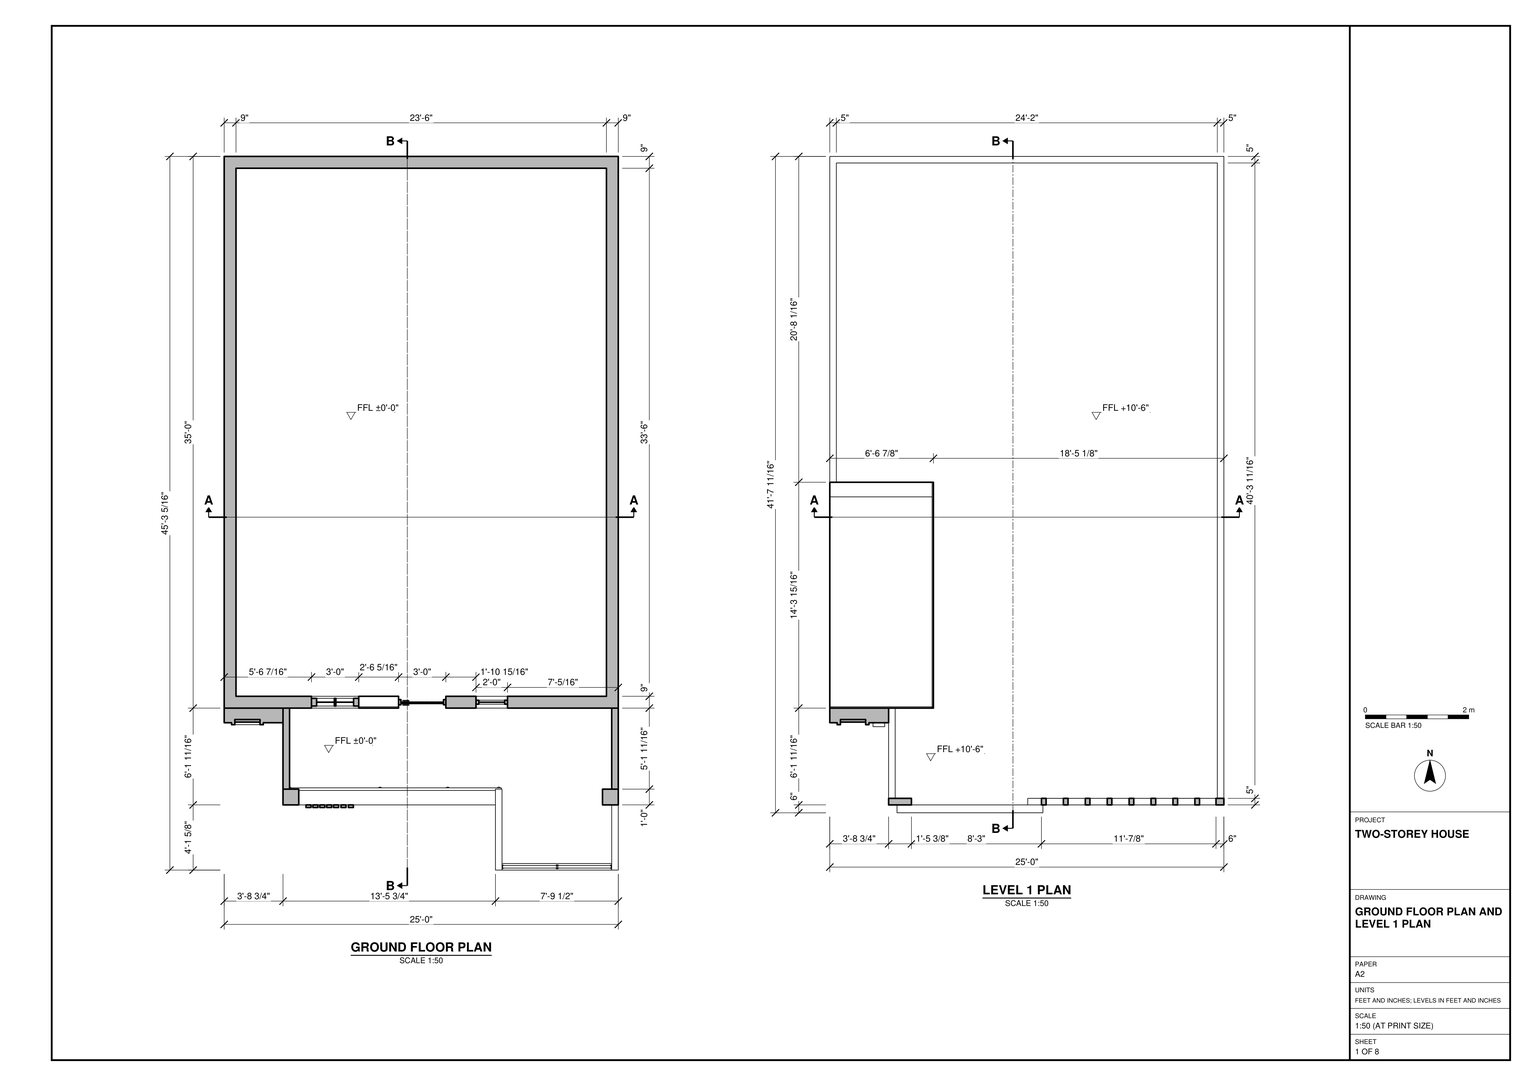
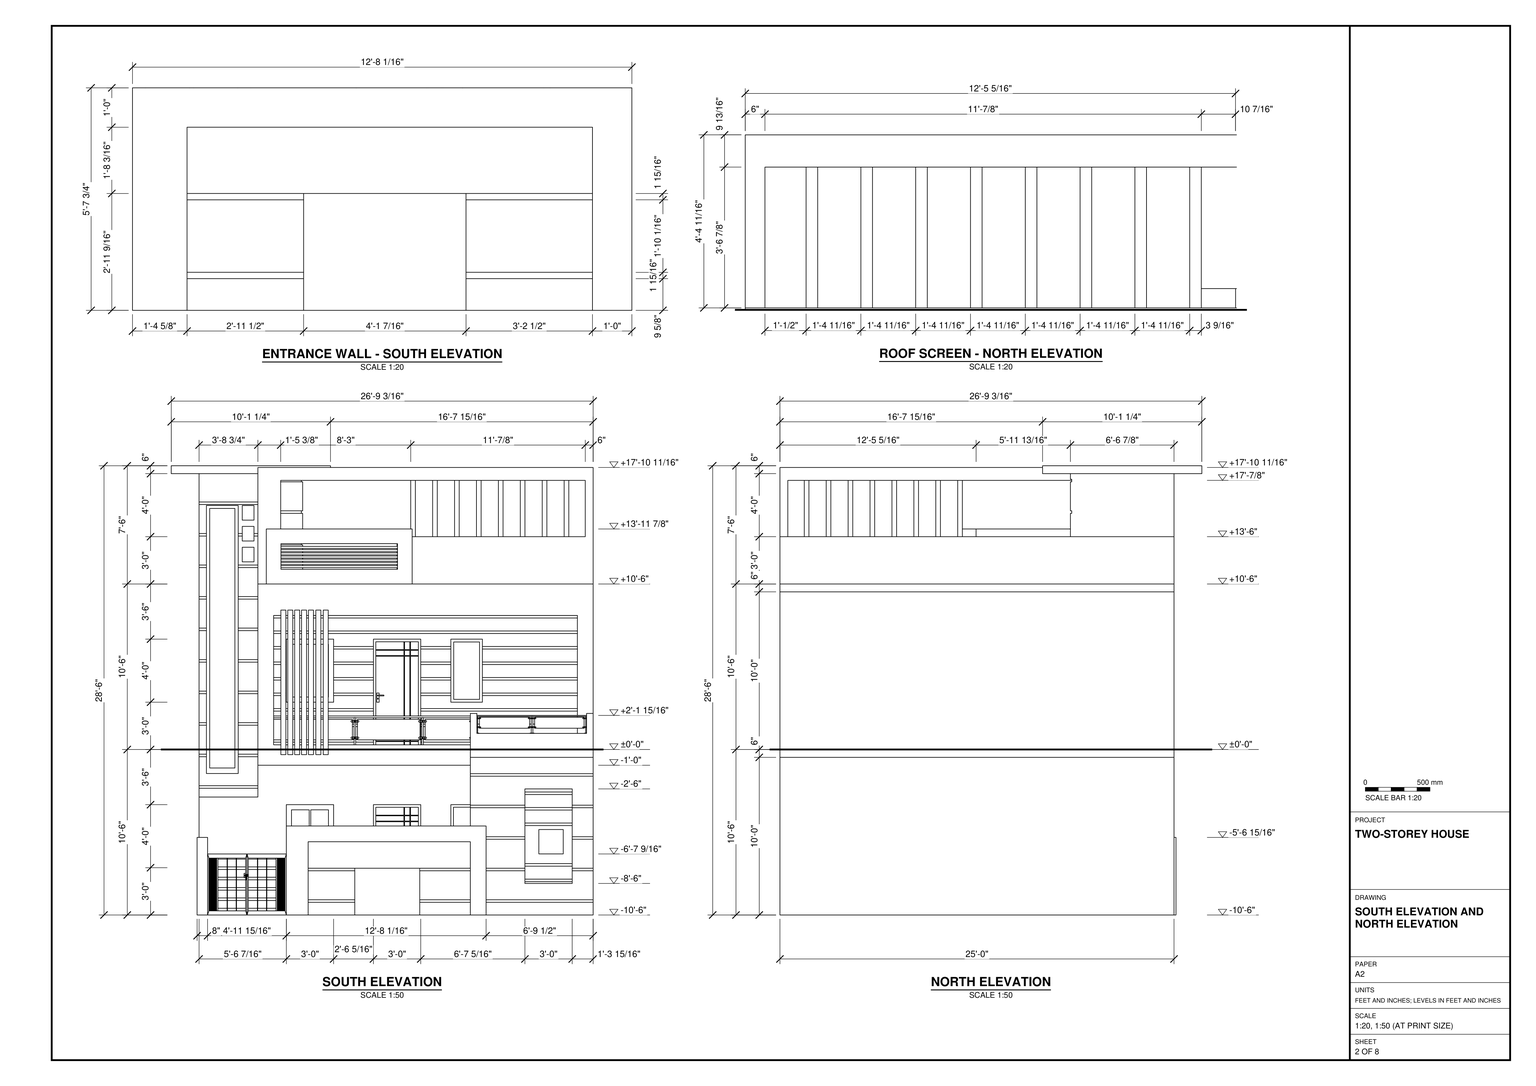
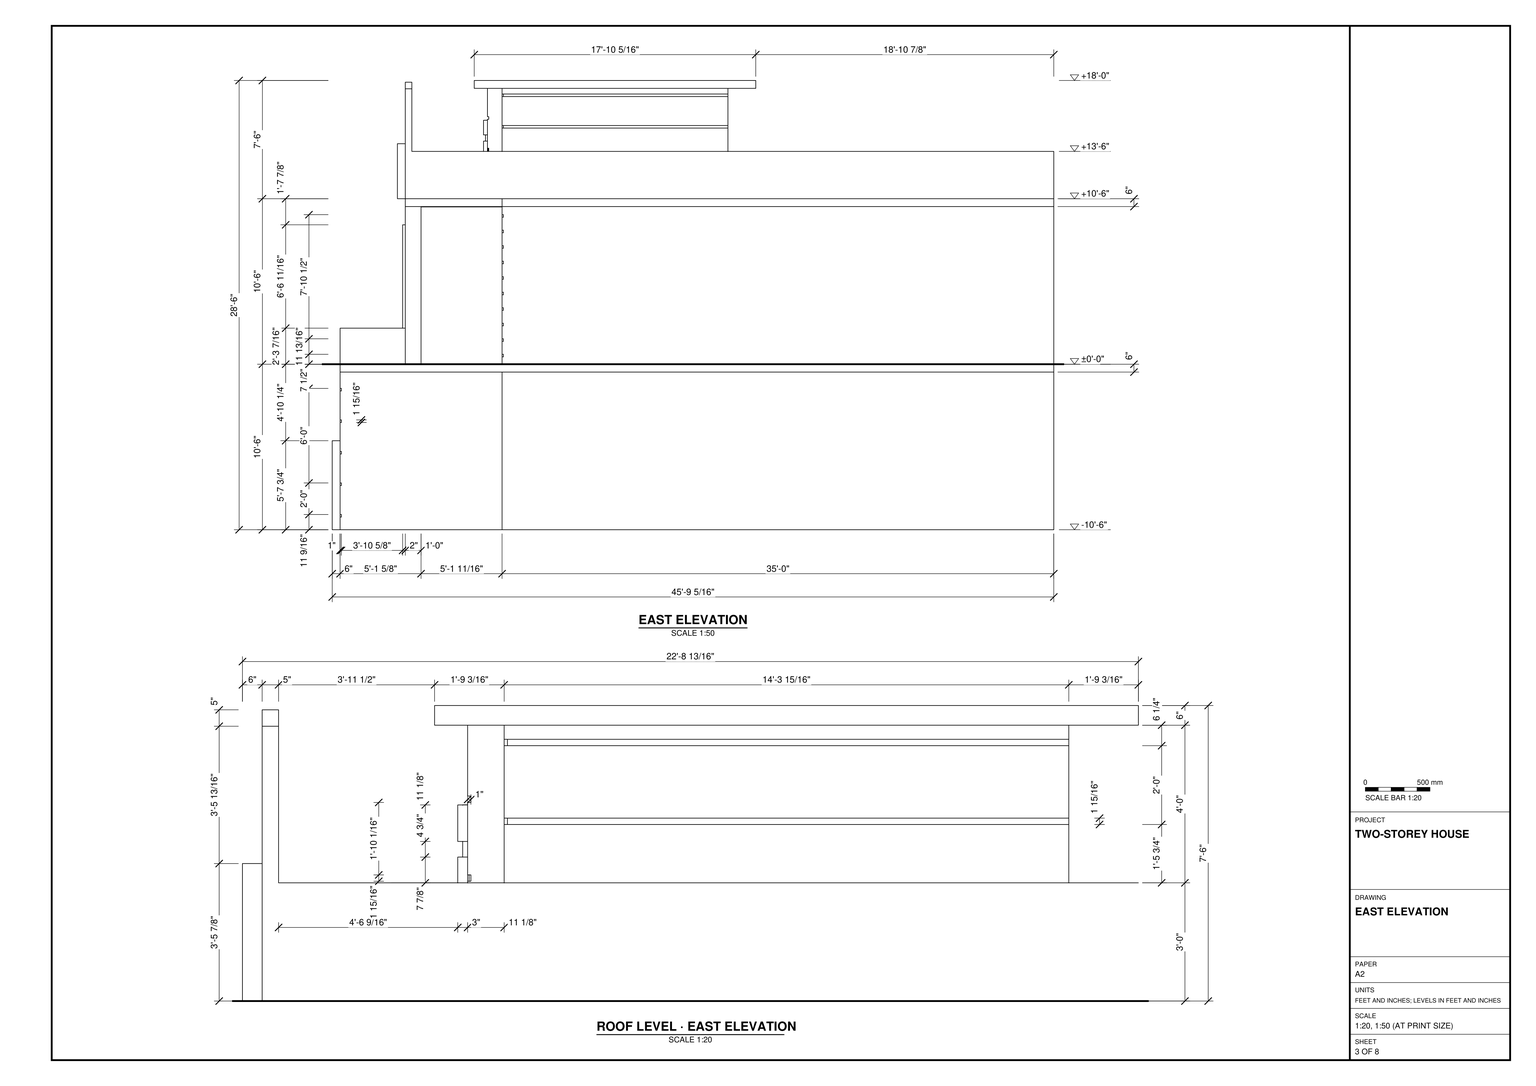
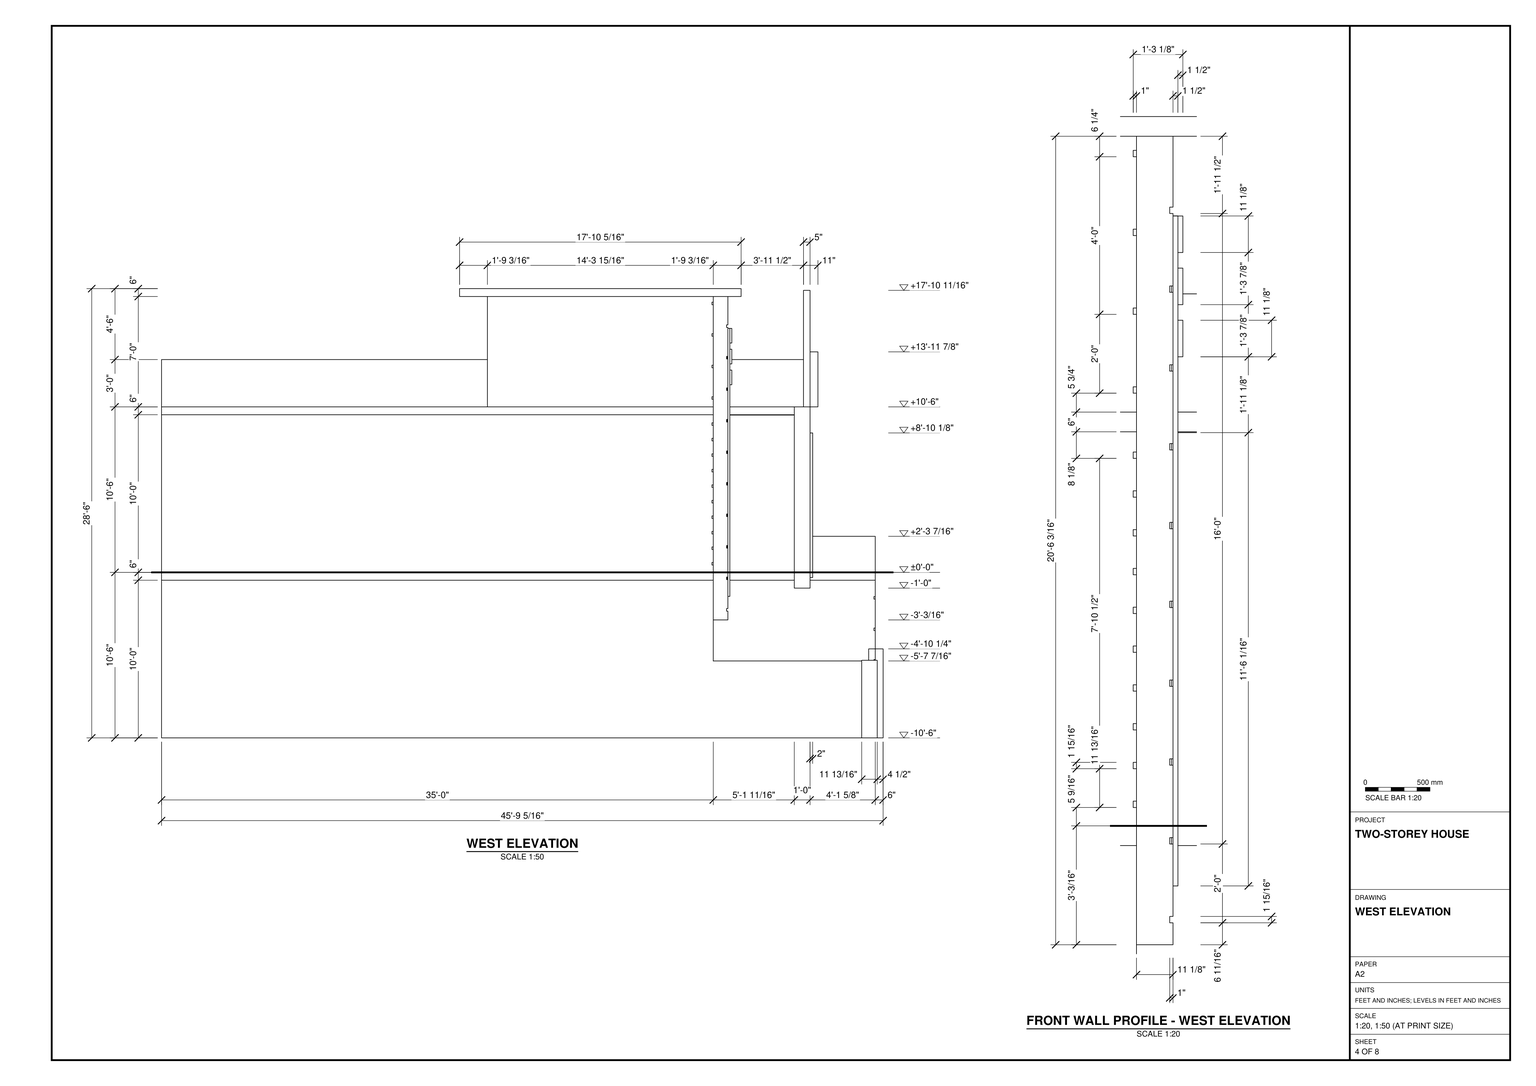
Build the two-storey house in SketchUp from task_files/diagram_01.pdf. Work in feet and inches. Set the ground floor at ±0'-0" and the next storey at +10'-6". The overall model, including the front projections and roof overhang, is 26'-9 3/16" wide, 45'-9 5/16" deep and 28'-6" high.

Start with the 25'-0" by 35'-0" rectangular ground-floor block. Use the wall thicknesses shown in plan and the slab thicknesses shown in elevation. Build the stepped south frontage around the recessed door and window openings. At the lower entrance, place the gate beside the broad framed entrance wall. Above it, model the balcony with its low railing, the horizontal bands on the wall behind it, the tall narrow panel at the left and the row of vertical fins. Follow the plans and elevations for the flat roof, low terrace parapet, raised canopy and roof screen, distinguishing the upright screen members from the horizontal slats.

Use separate groups or components for the walls, slabs, roof and each furniture or joinery piece shown. Use components for repeated parts. Any decor or loose items shown may be represented by suitable library components. Save one SketchUp model as output_files/two_storey_house_with_a_screened_roof_terrace.skp.

# SketchUp Ruby script. Lengths in inches.
U = 1.inch
M = Sketchup.active_model
def pt(a) = Geom::Point3d.new(a.map { |v| v * U })
def face(e, loops, mat)
  f = e.add_face(loops[0].map { |a| pt(a) })
  loops[1..].each { |l| e.add_face(l.map { |a| pt(a) }).erase! }
  f.material = f.back_material = mat if mat
  f
end
# faces: each face lists its corners as indices into pts; further lists are holes
def faces(e, pts, list, mat = nil) = list.each { |f| face(e, (f[0].is_a?(Array) ? f : [f]).map { |l| l.map { |i| pts[i] } }, mat) }
# xy, xz, yz: faces in a plane at the given z, y or x. An outline is a flat list of corners, or four numbers for a rectangle; further outlines are holes
def ring(l) = l.size == 4 ? [[l[0], l[1]], [l[2], l[1]], [l[2], l[3]], [l[0], l[3]]] : l.each_slice(2).to_a
def flat(e, list, mat, &to3) = list.each { |f| face(e, (f[0].is_a?(Array) ? f : [f]).map { |l| ring(l).map { |u, v| to3.(u, v) } }, mat) }
def xy(e, z, list, mat = nil) = flat(e, list, mat) { |x, y| [x, y, z] }
def xz(e, y, list, mat = nil) = flat(e, list, mat) { |x, z| [x, y, z] }
def yz(e, x, list, mat = nil) = flat(e, list, mat) { |y, z| [x, y, z] }
def lines(e, pts, list) = list.each { |a, b| e.add_line(pt(pts[a]), pt(pts[b])) }
# prism: a flat outline (further loops are holes) pulled along v
def prism(e, loops, v, mat = nil)
  f = face(e, loops, mat); d = Geom::Vector3d.new(v.map { |x| x * U })
  f.pushpull(f.normal.samedirection?(d) ? d.length : -d.length)
end
def box(e, o, s, mat = nil) = prism(e, [[o, [o[0] + s[0], o[1], o[2]], [o[0] + s[0], o[1] + s[1], o[2]], [o[0], o[1] + s[1], o[2]]]], [0, 0, s[2]], mat)
def at(x, y, z, deg = 0) = Geom::Transformation.translation(pt([x, y, z])) * Geom::Transformation.rotation(ORIGIN, Z_AXIS, deg.degrees)
def axes(o, x, y, z) = Geom::Transformation.new([*x, 0, *y, 0, *z, 0, *pt(o).to_a, 1])
def part(name) = M.definitions.add(name)
# library, detail: a bought-in or finely detailed component or shape, given as its bounding box
def library(name, o, s) = part(name).tap { |d| box(d.entities, o, s) }
def detail(e, o, s) = box(e.add_group.entities, o, s)
def put(e, d, t, mat = nil) = e.add_instance(d, t).tap { |i| i.material = mat if mat }
def group(e, t, mat = nil) = e.add_group.tap { |g| g.transformation = t; g.material = mat if mat }.entities
root = M.entities
M.materials.add("[Blacktop Old 02]").color = [143, 145, 145]
M.materials.add("[Color A01]").color = [255, 204, 204]
M.materials.add("[Color B03]").color = [255, 140, 101]
M.materials.add("[Color C03]").color = [255, 178, 101]
M.materials.add("[Color E05]").color = [255, 255, 0]
M.materials.add("[Color G02]").color = [153, 255, 153]
M.materials.add("[Color H06]").color = [0, 204, 204]
M.materials.add("[Color M00]").color = [255, 255, 255]
M.materials.add("[Color M05]").color = [114, 114, 114]
M.materials.add("[Color M09]").color = [0, 0, 0]
M.materials.add("[Formica Beige]").color = [211, 187, 149]
M.materials.add("[Translucent Glass Blue]").color = [100, 149, 237]
M.materials["[Translucent Glass Blue]"].alpha = 0.5
M.materials.add("[Wood Cherry Original]").color = [152, 86, 42]
c1 = library("Untitled",[0,0,0],[36,4.39,84])
c2 = library("Untitled\#1",[131.66,19.68,0],[2.41,197.25,46.46])
c3 = part("Group4\#2")
xy(c3.entities,0,[[-14.0625,-20.0625,-0.59,20.0625],[0.59,-20.0625,14.0625,20.0625]])
c4 = part("Group3\#1")
prism(c4.entities,[[[-18,24,0],[18,24,0],[18,-24,0],[-18,-24,0]],[[0.59,20.0625,0],[0.59,-20.0625,0],[14.0625,-20.0625,0],[14.0625,20.0625,0]],[[-0.59,20.0625,0],[-14.0625,20.0625,0],[-14.0625,-20.0625,0],[-0.59,-20.0625,0]]],[0,0,5.875])
put(c4.entities,c3,at(0,0,2.9375),"[Translucent Glass Blue]")
c5 = part("Group\#15")
box(c5.entities,[0,0,0],[3.8125,110.0625,2],"[Wood Cherry Original]")
c6 = part("Group\#6")
box(c6.entities,[0,0,0],[8.9375,11.125,3])
c7 = part("Group22\#1")
xy(c7.entities,126,[[295,-61.6875,300,0]])
xy(c7.entities,246,[[295,-61.6875,300,0]])
xz(c7.entities,-61.6875,[[295,126,300,246]])
xz(c7.entities,0,[[295,126,300,246]])
yz(c7.entities,295,[[-61.6875,126,0,246]])
yz(c7.entities,300,[[-61.6875,126,0,246]],"[Color M00]")
c8 = part("Group21\#1")
xy(c8.entities,126,[[206.5,-123.3125,211.5,-61.6875],[211.5,-123.3125,211.5,-118.3125,295,-118.3125,295,-73.6875,300,-73.6875,300,-123.3125]])
xy(c8.entities,138.25,[[211.5,-123.3125,295,-118.3125]])
xy(c8.entities,153.4375,[[206.5,-123.3125,211.5,-61.6875],[295,-123.3125,300,-73.6875]])
xz(c8.entities,-123.3125,[[206.5,126,300,126,300,153.4375,295,153.4375,295,138.25,211.5,138.25,211.5,153.4375,206.5,153.4375]])
xz(c8.entities,-118.3125,[[211.5,126,295,138.25]])
xz(c8.entities,-73.6875,[[295,126,300,153.4375]])
xz(c8.entities,-61.6875,[[206.5,126,211.5,153.4375]])
yz(c8.entities,206.5,[[-123.3125,126,-61.6875,153.4375]])
yz(c8.entities,211.5,[[-118.3125,126,-61.6875,153.4375],[-123.3125,138.25,-118.3125,153.4375]])
yz(c8.entities,295,[[-118.3125,126,-118.3125,138.25,-123.3125,138.25,-123.3125,153.4375,-73.6875,153.4375,-73.6875,126]])
yz(c8.entities,300,[[-123.3125,126,-73.6875,153.4375]])
c9 = part("Group22\#2")
box(c9.entities,[295,-61.6875,126],[5,61.6875,120])
c10 = library("Group\#9",[0,0,0],[87.4375,3.15,36.98])
c11 = library("Group\#10",[0,0,0],[163.16,3.15,36.98])
c12 = part("Group\#16")
box(c12.entities,[0,0,0],[2.53,1.5625,88.69])
c13 = part("Group\#17")
box(c13.entities,[0,0,0],[3.53,5,42.875])
c14 = part("Group31\#1")
xy(c14.entities,252,[[150.6875,-73.6875,150.6875,-68.6875,295,-68.6875,295,415,5,415,5,171.9375,0,171.9375,0,420,300,420,300,-73.6875],[44.78,-73.6875,62.15,-68.6875]])
xy(c14.entities,252,[[51.1875,-79.6875,150.6875,-73.6875],[150.6875,-79.6875,162.23,-73.6875]],"[Color G02]")
xy(c14.entities,263.17,[[150.6875,-79.6875,151.05,-73.6875]])
xy(c14.entities,263.17,[[62.36,-79.6875,150.6875,-73.6875]],"[Color G02]")
xy(c14.entities,282.7,[[62.36,-79.6875,151.05,-73.6875]],"[Color G02]")
xy(c14.entities,288,[[150.6875,-73.6875,277.9375,-68.6875],[281.47,-73.6875,294,-68.6875]])
xy(c14.entities,288,[[295,-68.6875,300,-68.6875,300,420,0,420,0,171.9375,5,171.9375,5,415,295,415]],"[Color M00]")
xy(c14.entities,293.875,[[51.1875,-79.6875,162.23,-73.6875]],"[Color G02]")
xy(c14.entities,330.875,[[62.15,-73.6875,294,-68.6875]])
xy(c14.entities,340.6875,[[44.78,-73.6875,300,-68.6875]])
xz(c14.entities,-79.6875,[[[51.1875,252,162.23,293.875],[62.36,263.17,151.05,282.7]]],"[Color G02]")
xz(c14.entities,-73.6875,[[44.78,252,51.1875,252,51.1875,293.875,62.15,293.875,62.15,330.875,294,330.875,294,288,162.23,288,162.23,252,300,252,300,340.6875,44.78,340.6875],[51.1875,252,62.15,293.875],[150.6875,252,150.6875,263.17,151.05,263.17,151.05,282.7,150.6875,282.7,150.6875,288,162.23,288,162.23,252],[150.6875,263.17,151.05,282.7],[150.6875,288,162.23,293.875]])
xz(c14.entities,-73.6875,[[62.15,252,62.15,293.875,150.6875,293.875,150.6875,282.7,62.36,282.7,62.36,263.17,150.6875,263.17,150.6875,252]],"[Color G02]")
xz(c14.entities,-68.6875,[[44.78,252,44.78,340.6875,300,340.6875,300,288,294,288,294,330.875,62.15,330.875,62.15,252]])
xz(c14.entities,-68.6875,[[150.6875,252,295,288]],"[Formica Beige]")
xz(c14.entities,171.9375,[[0,252,5,288]])
xz(c14.entities,415,[[5,252,295,288]],"[Color M00]")
xz(c14.entities,420,[[0,252,300,288]],"[Color M00]")
yz(c14.entities,0,[[171.9375,252,420,288]],"[Color M00]")
yz(c14.entities,5,[[171.9375,252,415,288]],"[Color M00]")
yz(c14.entities,44.78,[[-73.6875,252,-68.6875,340.6875]])
yz(c14.entities,51.1875,[[-79.6875,252,-73.6875,293.875]],"[Color G02]")
yz(c14.entities,62.15,[[-73.6875,252,-68.6875,330.875]])
yz(c14.entities,62.36,[[-79.6875,263.17,-73.6875,282.7]],"[Color G02]")
yz(c14.entities,150.6875,[[-73.6875,252,-68.6875,288]])
yz(c14.entities,151.05,[[-79.6875,263.17,-73.6875,282.7]],"[Color G02]")
yz(c14.entities,162.23,[[-79.6875,252,-73.6875,293.875]],"[Color G02]")
yz(c14.entities,294,[[-73.6875,288,-68.6875,330.875]])
yz(c14.entities,295,[[-68.6875,252,415,288]],"[Color M00]")
yz(c14.entities,300,[[-73.6875,335.6875,-68.6875,340.6875]])
yz(c14.entities,300,[[-73.6875,252,420,252,420,288,-68.6875,288,-68.6875,335.6875,-73.6875,335.6875]],"[Color M00]")
p = [[295,-73.6875,335.6875],[295,-68.6875,335.6875]]
lines(c14.entities,p,[[0,1]])
put(c14.entities,c12,axes([62.36,-78.14,279.05],[0,1,0],[0,0,1],[1,0,0]),"[Color M05]")
put(c14.entities,c12,axes([62.36,-78.14,276.61],[0,1,0],[0,0,1],[1,0,0]),"[Color M05]")
put(c14.entities,c12,axes([62.36,-78.14,274.17],[0,1,0],[0,0,1],[1,0,0]),"[Color M05]")
put(c14.entities,c12,axes([62.36,-78.14,271.74],[0,1,0],[0,0,1],[1,0,0]),"[Color M05]")
put(c14.entities,c12,axes([62.36,-78.14,269.3],[0,1,0],[0,0,1],[1,0,0]),"[Color M05]")
put(c14.entities,c12,axes([62.36,-78.14,266.86],[0,1,0],[0,0,1],[1,0,0]),"[Color M05]")
put(c14.entities,c12,axes([62.36,-78.14,264.42],[0,1,0],[0,0,1],[1,0,0]),"[Color M05]")
put(c14.entities,c12,axes([62.36,-78.14,259.55],[0,1,0],[0,0,1],[1,0,0]))
put(c14.entities,c12,axes([62.36,-78.14,257.11],[0,1,0],[0,0,1],[1,0,0]))
put(c14.entities,c13,at(277.9375,-73.6875,288))
put(c14.entities,c13,at(161.125,-73.6875,288))
put(c14.entities,c13,at(177.8125,-73.6875,288))
put(c14.entities,c13,at(194.5,-73.6875,288))
put(c14.entities,c13,at(211.1875,-73.6875,288))
put(c14.entities,c13,at(227.875,-73.6875,288))
put(c14.entities,c13,at(244.5625,-73.6875,288))
put(c14.entities,c13,at(261.25,-73.6875,288))
c15 = part("Group32\#1")
prism(c15.entities,[[[44.78,0,288.02],[44.78,0,252.02],[44.78,-68.6875,252],[44.78,-68.6875,288]]],[5,0,0])
xy(root,36,[[212.875,132.3125,236.875,135.3125]])
xy(root,37.96,[[214.83,132.3125,234.92,133.8125],[214.83,133.8125,234.92,135.3125]],"[Color M09]")
xy(root,82.04,[[214.83,132.3125,234.92,133.8125],[214.83,133.8125,234.92,135.3125]],"[Color M09]")
xy(root,84,[[212.875,132.3125,236.875,135.3125]])
xy(root,89.79,[[21.1875,118.1875,65.96,129.3125]])
xy(root,96.48,[[21.1875,118.1875,65.96,119.1875]],"[Color G02]")
xy(root,98.42,[[21.1875,118.1875,65.96,119.1875]],"[Color G02]")
xy(root,107.71,[[26.79,116.6875,50.99,118.1875]])
xy(root,111.9,[[29.3,116.6875,48.48,118.66],[29.3,118.66,48.48,120.625]])
xy(root,120.48,[[21.1875,118.1875,26.79,119.1875],[50.99,118.1875,65.96,119.1875]],"[Color G02]")
xy(root,122.42,[[21.1875,118.1875,26.79,119.1875],[50.99,118.1875,65.96,119.1875]],"[Color G02]")
xy(root,144.48,[[21.1875,118.1875,26.79,119.1875],[50.99,118.1875,65.96,119.1875]],"[Color G02]")
xy(root,146.42,[[21.1875,118.1875,26.79,119.1875],[50.99,118.1875,65.96,119.1875]],"[Color G02]")
xy(root,162,[[212.875,132.3125,236.875,135.3125]])
xy(root,164.17,[[215.04,132.3125,234.71,133.8125],[215.04,133.8125,234.71,135.3125]],"[Color M09]")
xy(root,168.48,[[21.1875,118.1875,26.79,119.1875],[50.99,118.1875,65.96,119.1875]],"[Color G02]")
xy(root,170.42,[[21.1875,118.1875,26.79,119.1875],[50.99,118.1875,65.96,119.1875]],"[Color G02]")
xy(root,192.48,[[21.1875,118.1875,26.79,119.1875],[50.99,118.1875,65.96,119.1875]],"[Color G02]")
xy(root,194.42,[[21.1875,118.1875,26.79,119.1875],[50.99,118.1875,65.96,119.1875]],"[Color G02]")
xy(root,207.83,[[215.04,132.3125,234.71,133.8125],[215.04,133.8125,234.71,135.3125]],"[Color M09]")
xy(root,210,[[212.875,132.3125,236.875,135.3125]])
xy(root,216.48,[[21.1875,118.1875,26.79,119.1875],[50.99,118.1875,65.96,119.1875]],"[Color G02]")
xy(root,218.42,[[21.1875,118.1875,26.79,119.1875],[50.99,118.1875,65.96,119.1875]],"[Color G02]")
xy(root,240.48,[[21.1875,118.1875,26.79,119.1875],[50.99,118.1875,65.96,119.1875]],"[Color G02]")
xy(root,242.42,[[21.1875,118.1875,26.79,119.1875],[50.99,118.1875,65.96,119.1875]],"[Color G02]")
xy(root,264.48,[[21.1875,118.1875,26.79,119.1875],[50.99,118.1875,65.96,119.1875]],"[Color G02]")
xy(root,266.42,[[21.1875,118.1875,26.79,119.1875],[50.99,118.1875,65.96,119.1875]],"[Color G02]")
xy(root,288.48,[[21.1875,118.1875,26.79,119.1875],[50.99,118.1875,65.96,119.1875]],"[Color G02]")
xy(root,290.42,[[21.1875,118.1875,26.79,119.1875],[50.99,118.1875,65.96,119.1875]],"[Color G02]")
xy(root,309.52,[[29.3,116.6875,48.48,118.66],[29.3,118.66,48.48,120.625]])
xy(root,311.76,[[26.79,116.6875,50.99,118.1875]])
xy(root,312.48,[[21.1875,118.1875,65.96,119.1875]],"[Color G02]")
xy(root,314.42,[[21.1875,118.1875,65.96,119.1875]],"[Color G02]")
xy(root,336,[[21.1875,118.1875,65.96,129.3125]],"[Color G02]")
xz(root,116.6875,[[[26.79,107.71,50.99,311.76],[29.3,111.9,48.48,309.52]]])
xz(root,118.1875,[[21.1875,89.79,65.96,96.48],[21.1875,98.42,65.96,98.42,65.96,120.48,50.99,120.48,50.99,107.71,26.79,107.71,26.79,120.48,21.1875,120.48],[21.1875,122.42,26.79,144.48],[50.99,122.42,65.96,144.48],[21.1875,146.42,26.79,168.48],
  [50.99,146.42,65.96,168.48],[21.1875,170.42,26.79,192.48],[50.99,170.42,65.96,192.48],[21.1875,194.42,26.79,216.48],[50.99,194.42,65.96,216.48],
  [21.1875,218.42,26.79,240.48],[50.99,218.42,65.96,240.48],[21.1875,242.42,26.79,264.48],[50.99,242.42,65.96,264.48],[21.1875,266.42,26.79,288.48],
  [50.99,266.42,65.96,288.48],[21.1875,290.42,26.79,290.42,26.79,311.76,50.99,311.76,50.99,290.42,65.96,290.42,65.96,312.48,21.1875,312.48],[21.1875,314.42,65.96,336]],"[Color G02]")
xz(root,118.66,[[29.3,111.9,48.48,309.52]],"[Translucent Glass Blue]")
xz(root,119.1875,[[21.1875,96.48,65.96,98.42],[21.1875,120.48,26.79,122.42],[50.99,120.48,65.96,122.42],[21.1875,144.48,26.79,146.42],[50.99,144.48,65.96,146.42],
  [21.1875,168.48,26.79,170.42],[50.99,168.48,65.96,170.42],[21.1875,192.48,26.79,194.42],[50.99,192.48,65.96,194.42],[21.1875,216.48,26.79,218.42],
  [50.99,216.48,65.96,218.42],[21.1875,240.48,26.79,242.42],[50.99,240.48,65.96,242.42],[21.1875,264.48,26.79,266.42],[50.99,264.48,65.96,266.42],
  [21.1875,288.48,26.79,290.42],[50.99,288.48,65.96,290.42],[21.1875,312.48,65.96,314.42]],"[Color G02]")
xz(root,120.625,[[29.3,111.9,48.48,309.52]])
xz(root,129.3125,[[21.1875,89.79,65.96,336]])
xz(root,132.3125,[[[212.875,36,236.875,84],[214.83,37.96,234.92,82.04]],[[212.875,162,236.875,210],[215.04,164.17,234.71,207.83]]],"[Color M09]")
xz(root,133.8125,[[214.83,37.96,234.92,82.04],[215.04,164.17,234.71,207.83]],"[Translucent Glass Blue]")
xz(root,135.3125,[[[212.875,36,236.875,84],[214.83,37.96,234.92,82.04]],[[212.875,162,236.875,210],[215.04,164.17,234.71,207.83]]],"[Color M09]")
yz(root,21.1875,[[118.1875,89.79,118.1875,96.48,119.1875,96.48,119.1875,98.42,118.1875,98.42,118.1875,120.48,119.1875,120.48,119.1875,122.42,118.1875,122.42,118.1875,144.48,119.1875,144.48,119.1875,146.42,118.1875,146.42,118.1875,168.48,119.1875,168.48,119.1875,170.42,118.1875,170.42,118.1875,192.48,119.1875,192.48,119.1875,194.42,118.1875,194.42,118.1875,216.48,119.1875,216.48,119.1875,218.42,118.1875,218.42,118.1875,240.48,119.1875,240.48,119.1875,242.42,118.1875,242.42,118.1875,264.48,119.1875,264.48,119.1875,266.42,118.1875,266.42,118.1875,288.48,119.1875,288.48,119.1875,290.42,118.1875,290.42,118.1875,312.48,119.1875,312.48,119.1875,314.42,118.1875,314.42,118.1875,336,129.3125,336,129.3125,89.79]],"[Color G02]")
yz(root,26.79,[[116.6875,107.71,118.1875,311.76]])
yz(root,29.3,[[116.6875,111.9,118.66,309.52],[118.66,111.9,120.625,309.52]])
yz(root,48.48,[[116.6875,111.9,118.66,309.52],[118.66,111.9,120.625,309.52]])
yz(root,50.99,[[116.6875,107.71,118.1875,311.76]])
yz(root,65.96,[[118.1875,89.79,129.3125,89.79,129.3125,246,118.1875,246,118.1875,242.42,119.1875,242.42,119.1875,240.48,118.1875,240.48,118.1875,218.42,119.1875,218.42,119.1875,216.48,118.1875,216.48,118.1875,194.42,119.1875,194.42,119.1875,192.48,118.1875,192.48,118.1875,170.42,119.1875,170.42,119.1875,168.48,118.1875,168.48,118.1875,146.42,119.1875,146.42,119.1875,144.48,118.1875,144.48,118.1875,122.42,119.1875,122.42,119.1875,120.48,118.1875,120.48,118.1875,98.42,119.1875,98.42,119.1875,96.48,118.1875,96.48],[118.1875,246,129.3125,246,129.3125,336,118.1875,336,118.1875,314.42,119.1875,314.42,119.1875,312.48,118.1875,312.48,118.1875,290.42,119.1875,290.42,119.1875,288.48,118.1875,288.48,118.1875,266.42,119.1875,266.42,119.1875,264.48,118.1875,264.48]],"[Color G02]")
yz(root,212.875,[[132.3125,36,135.3125,84],[132.3125,162,135.3125,210]])
yz(root,214.83,[[132.3125,37.96,133.8125,82.04],[133.8125,37.96,135.3125,82.04]],"[Color M09]")
yz(root,215.04,[[132.3125,164.17,133.8125,207.83],[133.8125,164.17,135.3125,207.83]],"[Color M09]")
yz(root,234.71,[[132.3125,164.17,133.8125,207.83],[133.8125,164.17,135.3125,207.83]],"[Color M09]")
yz(root,234.92,[[132.3125,37.96,133.8125,82.04],[133.8125,37.96,135.3125,82.04]],"[Color M09]")
yz(root,236.875,[[132.3125,36,135.3125,84],[132.3125,162,135.3125,210]])
p = [[87.625,133.8125,36],[87.625,133.8125,84],[123.625,133.8125,84],[123.625,133.8125,36]]
lines(root,p,[[0,1],[1,2],[2,3],[3,0]])
put(root,c1,at(153.9375,131.4,0))
put(root,c1,at(153.9375,131.4,126))
put(root,c2,axes([93.61,24.58,0],[0,-0.12,0],[-0.30387,0,0],[0,0,1]))
g1 = group(root,at(21.1875,129.3125,0))
xy(g1,0,[[0,-113,0,420,300,420,300,0,168.75,0,168.75,9,291,9,291,411,9,411,9,9,132.75,9,132.75,0,5,0,5,-113]])
xy(g1,0,[[-1.5,-124.8125,6.5,-113]],"[Color C03]")
xy(g1,36,[[66.4375,0,102.4375,9],[191.6875,0,215.6875,9]])
xy(g1,58.5625,[[0,-113,5,0]],"[Formica Beige]")
xy(g1,59.0625,[[-1.5,-124.8125,6.5,-113]],"[Color C03]")
xy(g1,84,[[66.4375,0,102.4375,9],[132.75,0,168.75,9],[191.6875,0,215.6875,9]])
xy(g1,120,[[[0,0,300,420],[9,9,291,411]]])
xz(g1,-124.8125,[[-1.5,0,6.5,59.0625]],"[Color C03]")
xz(g1,-113,[[0,0,5,58.5625]])
xz(g1,-113,[[-1.5,0,-1.5,59.0625,6.5,59.0625,6.5,0,5,0,5,58.5625,0,58.5625,0,0]],"[Color C03]")
xz(g1,0,[[[5,0,132.75,0,132.75,84,168.75,84,168.75,0,300,0,300,120,0,120,0,58.5625,5,58.5625],[66.4375,36,102.4375,84],[191.6875,36,215.6875,84]]],"[Color B03]")
xz(g1,9,[[[9,0,9,120,291,120,291,0,168.75,0,168.75,84,132.75,84,132.75,0],[66.4375,36,102.4375,84],[191.6875,36,215.6875,84]]])
xz(g1,411,[[9,0,291,120]])
xz(g1,420,[[0,0,300,120]],"[Color M00]")
yz(g1,-1.5,[[-124.8125,0,-113,59.0625]],"[Color C03]")
yz(g1,0,[[-113,0,-113,58.5625,0,58.5625,0,120,420,120,420,0]],"[Color M00]")
yz(g1,5,[[-113,0,0,58.5625]],"[Formica Beige]")
yz(g1,6.5,[[-124.8125,0,-113,59.0625]],"[Color C03]")
yz(g1,9,[[9,0,411,120]])
yz(g1,66.4375,[[0,36,9,84]])
yz(g1,102.4375,[[0,36,9,84]])
yz(g1,132.75,[[0,0,9,84]])
yz(g1,168.75,[[0,0,9,84]])
yz(g1,191.6875,[[0,36,9,84]])
yz(g1,215.6875,[[0,36,9,84]])
yz(g1,291,[[9,0,411,120]])
yz(g1,300,[[0,0,420,120]],"[Color M00]")
put(root,c4,axes([105.625,136.75,60],[1,0,0],[0,0,1],[0,-1,0]),"[Wood Cherry Original]")
g2 = group(root,at(21.1875,129.3125,120),"[Blacktop Old 02]")
prism(g2,[[[0,420,0],[300,420,0],[300,-123.3125,0],[206.5,-123.3125,0],[206.5,-61.6875,0],[44.78,-61.6875,0],[44.78,0,0],[0,0,0]]],[0,0,6])
p = [[44.78,0,0],[44.78,0,-0.6875]]
lines(g2,p,[[0,1]])
g3 = group(root,at(21.1875,129.3125,126),"[Color A01]")
xy(g3,0,[[0,0,0,420,300,420,300,0,168.75,0,168.75,9,291,9,291,411,9,411,9,9,132.75,9,132.75,0]],"[Formica Beige]")
xy(g3,5.59,[[0,0,132.75,1],[168.75,0,300,1]],"[Formica Beige]")
xy(g3,7.53,[[0,0,132.75,1],[168.75,0,300,1]],"[Formica Beige]")
xy(g3,17.4,[[168.75,0,300,1]],"[Color M00]")
xy(g3,17.4,[[0,0,132.75,1]],"[Formica Beige]")
xy(g3,19.34,[[0,0,132.75,1],[168.75,0,300,1]],"[Formica Beige]")
xy(g3,29.22,[[0,0,132.75,1],[168.75,0,300,1]],"[Formica Beige]")
xy(g3,31.15,[[0,0,132.75,1],[168.75,0,300,1]],"[Formica Beige]")
xy(g3,36,[[66.4375,0,102.4375,9],[191.6875,0,215.6875,9]],"[Formica Beige]")
xy(g3,41.03,[[0,0,66.4375,1],[102.4375,0,132.75,1],[168.75,0,191.6875,1],[215.6875,0,300,1]],"[Formica Beige]")
xy(g3,42.97,[[0,0,66.4375,1],[102.4375,0,132.75,1],[168.75,0,191.6875,1],[215.6875,0,300,1]],"[Formica Beige]")
xy(g3,52.84,[[215.6875,0,300,1]],"[Color H06]")
xy(g3,52.84,[[0,0,66.4375,1],[102.4375,0,132.75,1],[168.75,0,191.6875,1]],"[Formica Beige]")
xy(g3,54.78,[[215.6875,0,300,1]],"[Color H06]")
xy(g3,54.78,[[0,0,66.4375,1],[102.4375,0,132.75,1],[168.75,0,191.6875,1]],"[Formica Beige]")
xy(g3,64.65,[[215.6875,0,300,1]],"[Color H06]")
xy(g3,64.65,[[0,0,66.4375,1],[102.4375,0,132.75,1],[168.75,0,191.6875,1]],"[Formica Beige]")
xy(g3,66.59,[[0,0,66.4375,1],[102.4375,0,132.75,1],[168.75,0,191.6875,1],[215.6875,0,300,1]],"[Formica Beige]")
xy(g3,76.47,[[215.6875,0,300,1]],"[Color H06]")
xy(g3,76.47,[[0,0,66.4375,1],[102.4375,0,132.75,1],[168.75,0,191.6875,1]],"[Formica Beige]")
xy(g3,78.4,[[0,0,66.4375,1],[102.4375,0,132.75,1],[168.75,0,191.6875,1],[215.6875,0,300,1]],"[Formica Beige]")
xy(g3,84,[[66.4375,0,102.4375,9],[132.75,0,168.75,9],[191.6875,0,215.6875,9]],"[Formica Beige]")
xy(g3,88.28,[[0,0,300,1]],"[Formica Beige]")
xy(g3,90.22,[[0,0,300,1]],"[Formica Beige]")
xy(g3,100.09,[[0,0,300,1]],"[Color H06]")
xy(g3,102.03,[[0,0,300,1]],"[Color H06]")
xy(g3,111.9,[[0,0,300,1]],"[Color H06]")
xy(g3,113.84,[[0,0,300,1]],"[Color H06]")
xy(g3,120,[[[0,0,300,420],[9,9,291,411]]],"[Formica Beige]")
xz(g3,0,[[0,0,132.75,5.59],[168.75,0,300,5.59],[0,7.53,132.75,17.4],[168.75,7.53,300,17.4],[0,19.34,132.75,29.22],
  [168.75,19.34,300,29.22],[0,31.15,132.75,31.15,132.75,41.03,102.4375,41.03,102.4375,36,66.4375,36,66.4375,41.03,0,41.03],[168.75,31.15,300,31.15,300,41.03,215.6875,41.03,215.6875,36,191.6875,36,191.6875,41.03,168.75,41.03],[0,42.97,66.4375,52.84],[102.4375,42.97,132.75,52.84],
  [168.75,42.97,191.6875,52.84],[215.6875,42.97,300,52.84],[0,54.78,66.4375,64.65],[102.4375,54.78,132.75,64.65],[168.75,54.78,191.6875,64.65],
  [215.6875,54.78,300,64.65],[0,66.59,66.4375,76.47],[102.4375,66.59,132.75,76.47],[168.75,66.59,191.6875,76.47],[215.6875,66.59,300,76.47],
  [0,78.4,66.4375,78.4,66.4375,84,102.4375,84,102.4375,78.4,132.75,78.4,132.75,84,168.75,84,168.75,78.4,191.6875,78.4,191.6875,84,215.6875,84,215.6875,78.4,300,78.4,300,88.28,0,88.28],[0,90.22,300,100.09],[0,102.03,300,111.9],[0,113.84,300,120]],"[Color H06]")
xz(g3,1,[[0,5.59,132.75,7.53],[168.75,5.59,300,7.53],[0,17.4,132.75,19.34],[168.75,17.4,300,19.34],[0,29.22,132.75,31.15],
  [168.75,29.22,300,31.15],[0,41.03,66.4375,42.97],[102.4375,41.03,132.75,42.97],[168.75,41.03,191.6875,42.97],[215.6875,41.03,300,42.97],
  [0,52.84,66.4375,54.78],[102.4375,52.84,132.75,54.78],[168.75,52.84,191.6875,54.78],[215.6875,52.84,300,54.78],[0,64.65,66.4375,66.59],
  [102.4375,64.65,132.75,66.59],[168.75,64.65,191.6875,66.59],[215.6875,64.65,300,66.59],[0,76.47,66.4375,78.4],[102.4375,76.47,132.75,78.4],
  [168.75,76.47,191.6875,78.4],[215.6875,76.47,300,78.4],[0,88.28,300,90.22],[0,100.09,300,102.03],[0,111.9,300,113.84]],"[Color M00]")
xz(g3,9,[[[9,0,9,120,291,120,291,0,168.75,0,168.75,84,132.75,84,132.75,0],[66.4375,36,102.4375,84],[191.6875,36,215.6875,84]]],"[Formica Beige]")
xz(g3,411,[[9,0,291,120]],"[Formica Beige]")
xz(g3,420,[[0,0,300,120]],"[Color M00]")
yz(g3,0,[[0,0,0,5.59,1,5.59,1,7.53,0,7.53,0,17.4,1,17.4,1,19.34,0,19.34,0,29.22,1,29.22,1,31.15,0,31.15,0,41.03,1,41.03,1,42.97,0,42.97,0,52.84,1,52.84,1,54.78,0,54.78,0,64.65,1,64.65,1,66.59,0,66.59,0,76.47,1,76.47,1,78.4,0,78.4,0,88.28,1,88.28,1,90.22,0,90.22,0,100.09,1,100.09,1,102.03,0,102.03,0,111.9,1,111.9,1,113.84,0,113.84,0,120,420,120,420,0]],"[Color M00]")
yz(g3,0,[[0,5.59,1,7.53],[0,17.4,1,19.34],[0,29.22,1,31.15],[0,41.03,1,42.97],[0,52.84,1,54.78],
  [0,64.65,1,66.59],[0,76.47,1,78.4],[0,88.28,1,90.22],[0,100.09,1,102.03],[0,111.9,1,113.84]],"[Formica Beige]")
yz(g3,9,[[9,0,411,120]],"[Formica Beige]")
yz(g3,66.4375,[[0,36,9,36,9,84,0,84,0,78.4,1,78.4,1,76.47,0,76.47,0,66.59,1,66.59,1,64.65,0,64.65,0,54.78,1,54.78,1,52.84,0,52.84,0,42.97,1,42.97,1,41.03,0,41.03],[0,41.03,1,42.97],[0,52.84,1,54.78],[0,64.65,1,66.59],[0,76.47,1,78.4]],"[Formica Beige]")
yz(g3,102.4375,[[0,36,0,41.03,1,41.03,1,42.97,0,42.97,0,52.84,1,52.84,1,54.78,0,54.78,0,64.65,1,64.65,1,66.59,0,66.59,0,76.47,1,76.47,1,78.4,0,78.4,0,84,9,84,9,36],[0,41.03,1,42.97],[0,52.84,1,54.78],[0,64.65,1,66.59],[0,76.47,1,78.4]],"[Formica Beige]")
yz(g3,132.75,[[0,0,9,0,9,84,0,84,0,78.4,1,78.4,1,76.47,0,76.47,0,66.59,1,66.59,1,64.65,0,64.65,0,54.78,1,54.78,1,52.84,0,52.84,0,42.97,1,42.97,1,41.03,0,41.03,0,31.15,1,31.15,1,29.22,0,29.22,0,19.34,1,19.34,1,17.4,0,17.4,0,7.53,1,7.53,1,5.59,0,5.59],[0,5.59,1,7.53],[0,17.4,1,19.34],[0,29.22,1,31.15],[0,41.03,1,42.97],
  [0,52.84,1,54.78],[0,64.65,1,66.59],[0,76.47,1,78.4]],"[Formica Beige]")
yz(g3,168.75,[[0,0,0,5.59,1,5.59,1,7.53,0,7.53,0,17.4,1,17.4,1,19.34,0,19.34,0,29.22,1,29.22,1,31.15,0,31.15,0,41.03,1,41.03,1,42.97,0,42.97,0,52.84,1,52.84,1,54.78,0,54.78,0,64.65,1,64.65,1,66.59,0,66.59,0,76.47,1,76.47,1,78.4,0,78.4,0,84,9,84,9,0],[0,5.59,1,7.53],[0,17.4,1,19.34],[0,29.22,1,31.15],[0,41.03,1,42.97],
  [0,52.84,1,54.78],[0,64.65,1,66.59],[0,76.47,1,78.4]],"[Formica Beige]")
yz(g3,191.6875,[[0,36,9,36,9,84,0,84,0,78.4,1,78.4,1,76.47,0,76.47,0,66.59,1,66.59,1,64.65,0,64.65,0,54.78,1,54.78,1,52.84,0,52.84,0,42.97,1,42.97,1,41.03,0,41.03],[0,41.03,1,42.97],[0,52.84,1,54.78],[0,64.65,1,66.59],[0,76.47,1,78.4]],"[Formica Beige]")
yz(g3,215.6875,[[0,36,0,41.03,1,41.03,1,42.97,0,42.97,0,52.84,1,52.84,1,54.78,0,54.78,0,64.65,1,64.65,1,66.59,0,66.59,0,76.47,1,76.47,1,78.4,0,78.4,0,84,9,84,9,36],[0,41.03,1,42.97],[0,52.84,1,54.78],[0,64.65,1,66.59],[0,76.47,1,78.4]],"[Formica Beige]")
yz(g3,291,[[9,0,411,120]],"[Formica Beige]")
yz(g3,300,[[0,0,420,0,420,120,0,120,0,113.84,1,113.84,1,111.9,0,111.9,0,102.03,1,102.03,1,100.09,0,100.09,0,90.22,1,90.22,1,88.28,0,88.28,0,78.4,1,78.4,1,76.47,0,76.47,0,66.59,1,66.59,1,64.65,0,64.65,0,54.78,1,54.78,1,52.84,0,52.84,0,42.97,1,42.97,1,41.03,0,41.03,0,31.15,1,31.15,1,29.22,0,29.22,0,19.34,1,19.34,1,17.4,0,17.4,0,7.53,1,7.53,1,5.59,0,5.59]],"[Color M00]")
yz(g3,300,[[0,5.59,1,7.53],[0,17.4,1,19.34],[0,29.22,1,31.15],[0,41.03,1,42.97],[0,52.84,1,54.78],
  [0,64.65,1,66.59],[0,76.47,1,78.4],[0,88.28,1,90.22],[0,100.09,1,102.03],[0,111.9,1,113.84]],"[Formica Beige]")
put(root,c4,axes([105.625,136.75,186],[1,0,0],[0,0,1],[0,-1,0]),"[Wood Cherry Original]")
g4 = group(root,at(21.1875,129.3125,246),"[Blacktop Old 02]")
xy(g4,-132,[[44.78,-73.6875,206.5,-61.6875]],"[Color C03]")
xy(g4,-120,[[288,-73.6875,300,-61.6875]],"[Color C03]")
xy(g4,-116.4375,[[56.78,-73.6875,206.5,-61.6875]],"[Color C03]")
xy(g4,-18,[[56.78,-73.6875,288,-61.6875]],"[Color C03]")
xy(g4,0,[[0,0,300,420]])
xy(g4,0,[[44.78,-61.6875,300,0]],"[Color C03]")
xy(g4,6,[[44.78,-73.6875,300,-73.6875,300,420,0,420,0,160.8125,78.875,160.8125,78.875,0,44.78,0]],"[Color C03]")
xz(g4,-73.6875,[[44.78,-132,206.5,-132,206.5,-116.4375,56.78,-116.4375,56.78,-18,288,-18,288,-120,300,-120,300,6,44.78,6]],"[Color C03]")
xz(g4,-61.6875,[[44.78,-132,44.78,-18,56.78,-18,56.78,-116.4375,206.5,-116.4375,206.5,-132],[288,-120,300,0],[44.78,-18,288,0]],"[Color C03]")
xz(g4,0,[[0,0,44.78,6]])
xz(g4,420,[[0,0,300,6]])
yz(g4,0,[[0,0,420,6]])
yz(g4,44.78,[[-73.6875,-132,-61.6875,6],[-61.6875,0,0,6]],"[Color C03]")
yz(g4,56.78,[[-73.6875,-116.4375,-61.6875,-18]],"[Color C03]")
yz(g4,206.5,[[-73.6875,-132,-61.6875,-116.4375]],"[Color C03]")
yz(g4,288,[[-73.6875,-120,-61.6875,-18]],"[Color C03]")
yz(g4,300,[[0,0,420,6]])
yz(g4,300,[[-73.6875,0,0,6]],"[Color C03]")
yz(g4,300,[[-73.6875,-120,-61.6875,0]],"[Color M00]")
p = [[44.78,0,6.02],[44.78,0,6],[300,0,-18],[44.78,0,-18],[56.78,-73.6875,0],[56.78,-61.6875,0],
  [56.78,-61.6875,6],[288,-73.6875,0],[288,-61.6875,0]]
lines(g4,p,[[0,1],[2,3],[4,5],[6,5],[7,8]])
g5 = group(g4,at(0,11.125,6),"[Color G02]")
xy(g5,0,[[0,-11.125,78.875,160.8125]],"[Formica Beige]")
xy(g5,5.76,[[0,-11.125,78.875,-11.125,78.875,160.8125,77.875,160.8125,77.875,-10.125,0,-10.125]],"[Formica Beige]")
xy(g5,7.7,[[0,-11.125,77.875,-10.125],[77.875,-11.125,78.875,-10.125],[77.875,-10.125,78.875,160.8125]],"[Formica Beige]")
xy(g5,29.76,[[0,-11.125,78.875,-11.125,78.875,160.8125,77.875,160.8125,77.875,-10.125,0,-10.125]],"[Formica Beige]")
xy(g5,31.7,[[0,-11.125,77.875,-10.125],[77.875,-11.125,78.875,-10.125],[77.875,-10.125,78.875,160.8125]],"[Formica Beige]")
xy(g5,53.76,[[0,-11.125,78.875,-11.125,78.875,160.8125,77.875,160.8125,77.875,-10.125,0,-10.125]],"[Formica Beige]")
xy(g5,55.7,[[0,-11.125,77.875,-10.125],[77.875,-11.125,78.875,-10.125],[77.875,-10.125,78.875,160.8125]],"[Formica Beige]")
xy(g5,77.76,[[0,-11.125,78.875,-11.125,78.875,160.8125,77.875,160.8125,77.875,-10.125,0,-10.125]],"[Formica Beige]")
xy(g5,79.7,[[0,-11.125,77.875,-10.125],[77.875,-11.125,78.875,-10.125],[77.875,-10.125,78.875,160.8125]],"[Formica Beige]")
xy(g5,84,[[[-21.1875,-32.3125,100.0625,182],[0,-11.125,78.875,160.8125]],[0,-11.125,78.875,160.8125]],"[Formica Beige]")
xy(g5,90,[[-21.1875,-32.3125,100.0625,182]],"[Formica Beige]")
xz(g5,-32.3125,[[-21.1875,84,100.0625,90]],"[Formica Beige]")
xz(g5,-11.125,[[0,0,78.875,5.76],[0,7.7,78.875,29.76],[0,31.7,78.875,53.76],[0,55.7,78.875,77.76],[0,79.7,78.875,84]],"[Formica Beige]")
xz(g5,-10.125,[[0,5.76,77.875,7.7],[0,29.76,77.875,31.7],[0,53.76,77.875,55.7],[0,77.76,77.875,79.7]],"[Formica Beige]")
xz(g5,160.8125,[[0,0,0,84,78.875,84,78.875,79.7,77.875,79.7,77.875,77.76,78.875,77.76,78.875,55.7,77.875,55.7,77.875,53.76,78.875,53.76,78.875,31.7,77.875,31.7,77.875,29.76,78.875,29.76,78.875,7.7,77.875,7.7,77.875,5.76,78.875,5.76,78.875,0]],"[Formica Beige]")
xz(g5,182,[[-21.1875,84,100.0625,90]],"[Formica Beige]")
yz(g5,-21.1875,[[-32.3125,84,182,90]],"[Formica Beige]")
yz(g5,0,[[-11.125,0,-11.125,5.76,-10.125,5.76,-10.125,7.7,-11.125,7.7,-11.125,29.76,-10.125,29.76,-10.125,31.7,-11.125,31.7,-11.125,53.76,-10.125,53.76,-10.125,55.7,-11.125,55.7,-11.125,77.76,-10.125,77.76,-10.125,79.7,-11.125,79.7,-11.125,84,160.8125,84,160.8125,0],[-11.125,5.76,-10.125,7.7],[-11.125,29.76,-10.125,31.7],[-11.125,53.76,-10.125,55.7],[-11.125,77.76,-10.125,79.7]],"[Formica Beige]")
yz(g5,77.875,[[-10.125,5.76,160.8125,7.7],[-10.125,29.76,160.8125,31.7],[-10.125,53.76,160.8125,55.7],[-10.125,77.76,160.8125,79.7]],"[Formica Beige]")
yz(g5,78.875,[[-11.125,0,160.8125,5.76],[-11.125,7.7,160.8125,29.76],[-11.125,31.7,160.8125,53.76],[-11.125,55.7,160.8125,77.76],[-11.125,79.7,160.8125,84]],"[Formica Beige]")
yz(g5,100.0625,[[-32.3125,84,182,90]],"[Formica Beige]")
g6 = group(g4,at(62.28,-73.6875,-123.92),"[Wood Cherry Original]")
box(g6,[0,-2,0],[3.8125,2,110.0625],"[Wood Cherry Original]")
g7 = group(g4,at(67.53,-73.6875,-123.92),"[Wood Cherry Original]")
box(g7,[0,-2,0],[3.8125,2,110.0625],"[Wood Cherry Original]")
g8 = group(g4,at(72.78,-73.6875,-123.92))
box(g8,[0,-2,0],[3.8125,2,110.0625],"[Wood Cherry Original]")
g9 = group(g4,at(78.03,-73.6875,-123.92))
box(g9,[0,-2,0],[3.8125,2,110.0625],"[Wood Cherry Original]")
put(g4,c5,axes([83.28,-73.6875,-123.92],[1,0,0],[0,0,1],[0,-1,0]))
put(g4,c5,axes([88.91,-73.6875,-123.92],[1,0,0],[0,0,1],[0,-1,0]))
put(g4,c5,axes([94.53,-73.6875,-123.92],[1,0,0],[0,0,1],[0,-1,0]))
put(root,c6,axes([54.07,118.1875,300.6],[1,0,0],[0,0,1],[0,-1,0]))
put(root,c6,axes([54.07,118.1875,284.72],[1,0,0],[0,0,1],[0,-1,0]))
put(root,c6,axes([54.07,118.1875,268.85],[1,0,0],[0,0,1],[0,-1,0]))
g10 = group(root,at(65.96,67.625,246),"[Color C03]")
prism(g10,[[[0,61.6875,-0.25],[255.22,61.6875,-0.25],[255.22,0,-0.25],[0,0,-0.25],[0,50.5625,-0.25]]],[0,0,0.25])
g11 = group(root,at(227.6875,6,0),"[Color G02]")
xy(g11,0,[[-140.0625,0,-140.0625,5,0,5,0,123.3125,9,123.3125,9,9,84.5,9,84.5,123.3125,93.5,123.3125,93.5,0]])
xy(g11,0,[[-140.0625,-6,-123.45,0],[-87.95,-6,-38.5,0],[0,-6,12,0]],"[Color C03]")
xy(g11,9.65,[[-140.0625,0,93.5,1]])
xy(g11,11.59,[[-140.0625,0,93.5,1]])
xy(g11,24,[[41.5625,0,77.5625,7.25]])
xy(g11,25.35,[[41.5625,7.25,77.5625,8.25]],"[Color M00]")
xy(g11,27.29,[[41.5625,7.25,77.5625,8.25]])
xy(g11,33.65,[[-140.0625,0,41.5625,1],[77.5625,0,93.5,1]])
xy(g11,35.59,[[-140.0625,0,41.5625,1],[77.5625,0,93.5,1]])
xy(g11,35.59,[[-87.95,-6,-38.5,0]],"[Color C03]")
xy(g11,37.16,[[41.5625,7.25,77.5625,8.25]],"[Color M00]")
xy(g11,39.1,[[41.5625,7.25,77.5625,8.25]])
xy(g11,46.5,[[52.18,7.25,70.74,8.75]])
xy(g11,55.77,[[-123.45,-6,0,0]],"[Color C03]")
xy(g11,57.65,[[-140.0625,0,41.5625,1],[77.5625,0,93.5,1]])
xy(g11,59.59,[[-140.0625,0,41.5625,1],[77.5625,0,93.5,1]])
xy(g11,65.0625,[[52.18,7.25,70.74,8.75]])
xy(g11,67.77,[[-140.0625,0,0,5]])
xy(g11,67.77,[[-140.0625,-6,12,0]],"[Color C03]")
xy(g11,68.08,[[41.5625,7.25,77.5625,8.25]],"[Color M00]")
xy(g11,70.01,[[41.5625,7.25,77.5625,8.25]],"[Color M00]")
xy(g11,79.89,[[41.5625,7.25,77.5625,8.25]],"[Color M00]")
xy(g11,81.65,[[0,0,41.5625,1],[77.5625,0,93.5,1]])
xy(g11,81.83,[[41.5625,7.25,77.5625,8.25]],"[Color M00]")
xy(g11,83.59,[[0,0,41.5625,1],[77.5625,0,93.5,1]])
xy(g11,91.7,[[41.5625,7.25,77.5625,8.25]],"[Color M00]")
xy(g11,93.64,[[41.5625,7.25,77.5625,8.25]],"[Color M00]")
xy(g11,96,[[41.5625,0,77.5625,7.25]])
xy(g11,105.65,[[0,0,93.5,1]])
xy(g11,107.59,[[0,0,93.5,1]])
xy(g11,120,[[0,0,93.5,0,93.5,123.3125,84.5,123.3125,84.5,9,9,9,9,123.3125,0,123.3125]])
xz(g11,-6,[[-140.0625,0,-123.45,0,-123.45,55.77,0,55.77,0,0,12,0,12,67.77,-140.0625,67.77],[-87.95,0,-38.5,35.59]],"[Color C03]")
xz(g11,0,[[-140.0625,0,-123.45,9.65],[-123.45,0,-87.95,9.65],[-87.95,0,-38.5,9.65],[-38.5,0,0,9.65],[0,0,12,9.65],
  [12,0,93.5,9.65],[-140.0625,9.65,-123.45,11.59],[-123.45,9.65,-87.95,11.59],[-87.95,9.65,-38.5,11.59],[-38.5,9.65,0,11.59],
  [0,9.65,12,11.59],[12,9.65,93.5,11.59],[-140.0625,11.59,-123.45,33.65],[-123.45,11.59,-87.95,33.65],[-38.5,11.59,0,33.65],
  [0,11.59,12,33.65],[12,11.59,93.5,11.59,93.5,33.65,77.5625,33.65,77.5625,24,41.5625,24,41.5625,33.65,12,33.65],[-140.0625,33.65,-123.45,35.59],[-123.45,33.65,-87.95,35.59],[-87.95,33.65,-38.5,35.59],
  [-38.5,33.65,0,35.59],[0,33.65,12,35.59],[12,33.65,41.5625,35.59],[-140.0625,35.59,-123.45,55.77],[-123.45,35.59,0,55.77],
  [0,35.59,12,55.77],[12,35.59,41.5625,57.65],[77.5625,35.59,93.5,57.65],[-140.0625,55.77,-123.45,57.65],[-123.45,55.77,0,57.65],
  [0,55.77,12,57.65],[-140.0625,57.65,-123.45,59.59],[-123.45,57.65,0,59.59],[0,57.65,12,59.59],[12,57.65,41.5625,59.59],
  [-140.0625,59.59,-123.45,67.77],[-123.45,59.59,0,67.77],[0,59.59,12,67.77],[12,59.59,41.5625,59.59,41.5625,81.65,0,81.65,0,67.77,12,67.77],[77.5625,59.59,93.5,81.65],
  [0,83.59,41.5625,83.59,41.5625,96,77.5625,96,77.5625,83.59,93.5,83.59,93.5,105.65,0,105.65],[0,107.59,93.5,120]])
xz(g11,1,[[-140.0625,9.65,93.5,11.59],[-140.0625,33.65,41.5625,35.59],[77.5625,33.65,93.5,35.59],[-140.0625,57.65,41.5625,59.59],[77.5625,57.65,93.5,59.59],
  [0,81.65,41.5625,83.59],[77.5625,81.65,93.5,83.59],[0,105.65,93.5,107.59]])
xz(g11,5,[[-140.0625,0,0,67.77]])
xz(g11,7.25,[[41.5625,24,77.5625,25.35],[41.5625,27.29,77.5625,37.16],[41.5625,39.1,77.5625,46.5],[41.5625,46.5,52.18,46.5,52.18,65.0625,70.74,65.0625,70.74,46.5,77.5625,46.5,77.5625,68.08,41.5625,68.08],[41.5625,70.01,77.5625,79.89],
  [41.5625,81.83,77.5625,91.7],[41.5625,93.64,77.5625,96]],"[Color M00]")
xz(g11,8.25,[[41.5625,25.35,77.5625,27.29],[41.5625,37.16,77.5625,39.1],[41.5625,68.08,77.5625,70.01],[41.5625,79.89,77.5625,81.83],[41.5625,91.7,77.5625,93.64]],"[Color M00]")
xz(g11,8.75,[[52.18,46.5,70.74,65.0625]],"[Color E05]")
xz(g11,9,[[9,0,84.5,120]],"[Color M00]")
xz(g11,123.3125,[[0,0,9,120],[84.5,0,93.5,120]])
yz(g11,-140.0625,[[0,0,0,9.65,1,9.65,1,11.59,0,11.59,0,33.65,1,33.65,1,35.59,0,35.59,0,57.65,1,57.65,1,59.59,0,59.59,0,67.77,5,67.77,5,0],[0,9.65,1,11.59],[0,33.65,1,35.59],[0,57.65,1,59.59]])
yz(g11,-140.0625,[[-6,0,0,67.77]],"[Color C03]")
yz(g11,-123.45,[[-6,0,0,55.77]],"[Color C03]")
yz(g11,-87.95,[[-6,0,0,35.59]],"[Color C03]")
yz(g11,-38.5,[[-6,0,0,35.59]],"[Color C03]")
yz(g11,0,[[5,0,5,67.77,0,67.77,0,81.65,1,81.65,1,83.59,0,83.59,0,105.65,1,105.65,1,107.59,0,107.59,0,120,123.3125,120,123.3125,0],[0,81.65,1,83.59],[0,105.65,1,107.59]])
yz(g11,0,[[-6,0,0,55.77]],"[Color C03]")
yz(g11,9,[[9,0,123.3125,120]])
yz(g11,12,[[-6,0,0,67.77]],"[Color C03]")
yz(g11,41.5625,[[0,24,7.25,24,7.25,96,0,96,0,83.59,1,83.59,1,81.65,0,81.65,0,59.59,1,59.59,1,57.65,0,57.65,0,35.59,1,35.59,1,33.65,0,33.65],[0,33.65,1,35.59],[0,57.65,1,59.59],[0,81.65,1,83.59]])
yz(g11,52.18,[[7.25,46.5,8.75,65.0625]])
yz(g11,70.74,[[7.25,46.5,8.75,65.0625]])
yz(g11,77.5625,[[0,24,0,33.65,1,33.65,1,35.59,0,35.59,0,57.65,1,57.65,1,59.59,0,59.59,0,81.65,1,81.65,1,83.59,0,83.59,0,96,7.25,96,7.25,24],[0,33.65,1,35.59],[0,57.65,1,59.59],[0,81.65,1,83.59]])
yz(g11,84.5,[[9,0,123.3125,120]])
yz(g11,93.5,[[0,9.65,1,11.59],[0,33.65,1,35.59],[0,57.65,1,59.59],[0,81.65,1,83.59],[0,105.65,1,107.59]])
yz(g11,93.5,[[0,0,123.3125,0,123.3125,120,0,120,0,107.59,1,107.59,1,105.65,0,105.65,0,83.59,1,83.59,1,81.65,0,81.65,0,59.59,1,59.59,1,57.65,0,57.65,0,35.59,1,35.59,1,33.65,0,33.65,0,11.59,1,11.59,1,9.65,0,9.65]],"[Color M00]")
p = [[84.5,123.3125,0],[9,123.3125,0]]
lines(g11,p,[[0,1]])
put(root,c7,at(21.1875,129.3125,0),"[Formica Beige]")
put(root,c8,at(21.1875,129.3125,0))
put(root,c9,at(-229.04,129.3125,0),"[Formica Beige]")
put(root,c10,axes([230.72,6.93,138.25],[1,0,0],[0,1,0],[0,0,0.37]))
put(root,c11,axes([69,66.05,126],[1,0,0],[0,1,0],[0,0,0.69]))
put(root,c14,at(21.1875,129.3125,0))
put(root,c15,at(21.1875,129.3125,0),"[Color M00]")
